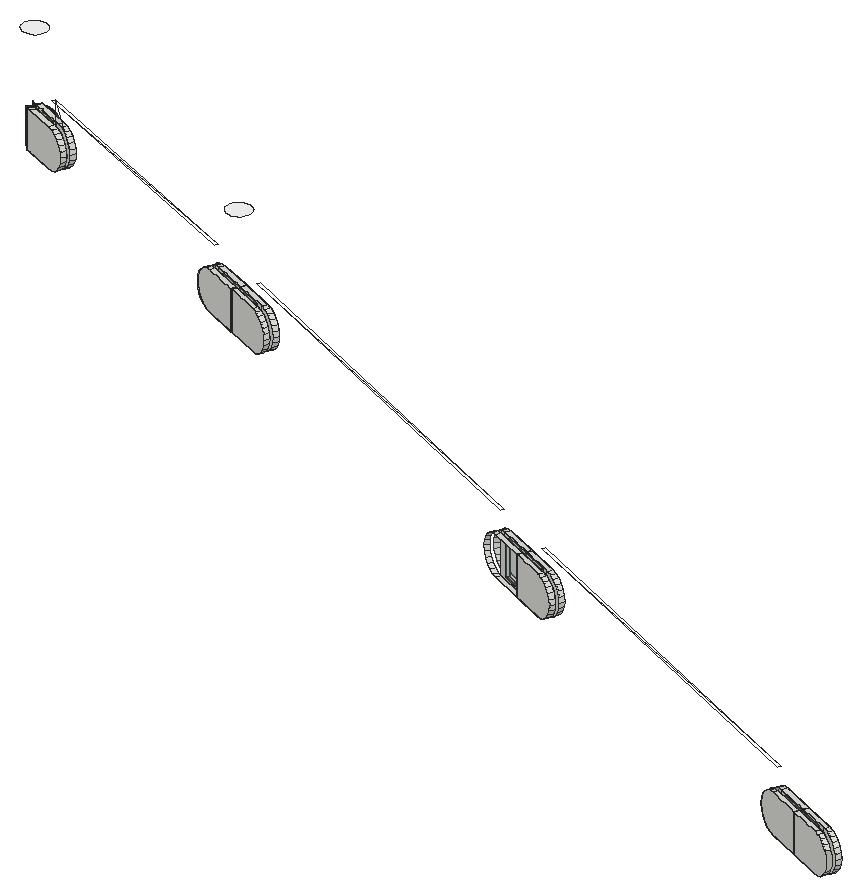
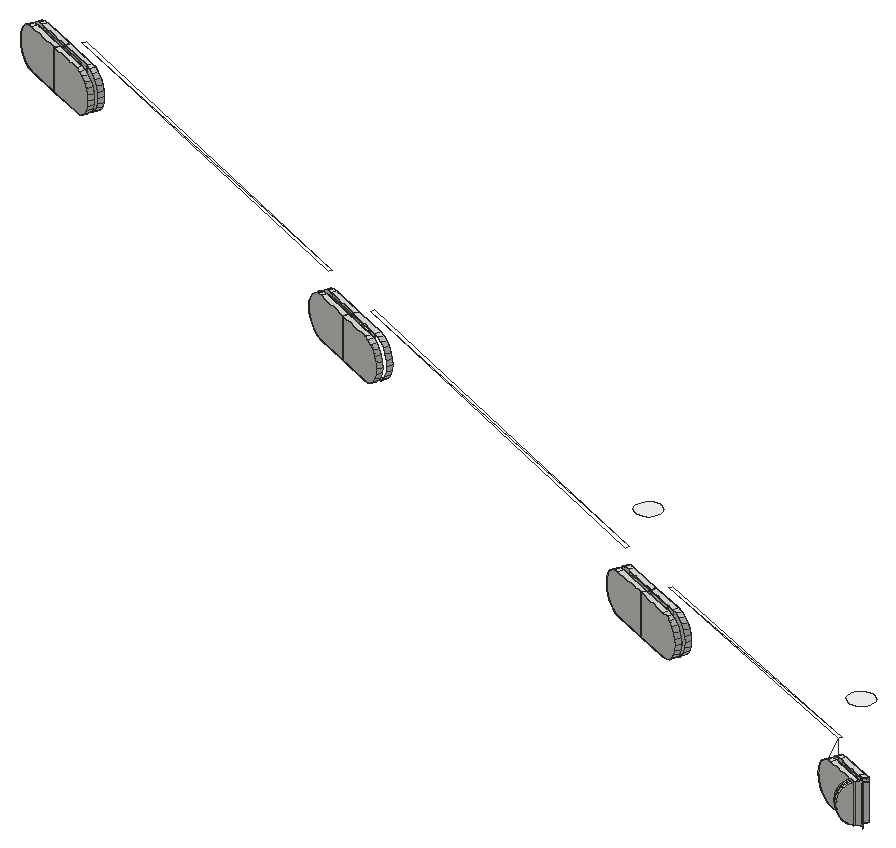
# SketchUp Ruby script. Lengths in inches.
U = 1.inch
M = Sketchup.active_model
def pt(a) = Geom::Point3d.new(a.map { |v| v * U })
def face(e, loops, mat)
  f = e.add_face(loops[0].map { |a| pt(a) })
  loops[1..].each { |l| e.add_face(l.map { |a| pt(a) }).erase! }
  f.material = f.back_material = mat if mat
  f
end
# faces: each face lists its corners as indices into pts; further lists are holes
def faces(e, pts, list, mat = nil) = list.each { |f| face(e, (f[0].is_a?(Array) ? f : [f]).map { |l| l.map { |i| pts[i] } }, mat) }
# xy, xz, yz: faces in a plane at the given z, y or x. An outline is a flat list of corners, or four numbers for a rectangle; further outlines are holes
def ring(l) = l.size == 4 ? [[l[0], l[1]], [l[2], l[1]], [l[2], l[3]], [l[0], l[3]]] : l.each_slice(2).to_a
def flat(e, list, mat, &to3) = list.each { |f| face(e, (f[0].is_a?(Array) ? f : [f]).map { |l| ring(l).map { |u, v| to3.(u, v) } }, mat) }
def xy(e, z, list, mat = nil) = flat(e, list, mat) { |x, y| [x, y, z] }
def xz(e, y, list, mat = nil) = flat(e, list, mat) { |x, z| [x, y, z] }
def yz(e, x, list, mat = nil) = flat(e, list, mat) { |y, z| [x, y, z] }
def lines(e, pts, list) = list.each { |a, b| e.add_line(pt(pts[a]), pt(pts[b])) }
# prism: a flat outline (further loops are holes) pulled along v
def prism(e, loops, v, mat = nil)
  f = face(e, loops, mat); d = Geom::Vector3d.new(v.map { |x| x * U })
  f.pushpull(f.normal.samedirection?(d) ? d.length : -d.length)
end
def box(e, o, s, mat = nil) = prism(e, [[o, [o[0] + s[0], o[1], o[2]], [o[0] + s[0], o[1] + s[1], o[2]], [o[0], o[1] + s[1], o[2]]]], [0, 0, s[2]], mat)
def at(x, y, z, deg = 0) = Geom::Transformation.translation(pt([x, y, z])) * Geom::Transformation.rotation(ORIGIN, Z_AXIS, deg.degrees)
def axes(o, x, y, z) = Geom::Transformation.new([*x, 0, *y, 0, *z, 0, *pt(o).to_a, 1])
def part(name) = M.definitions.add(name)
# library, detail: a bought-in or finely detailed component or shape, given as its bounding box
def library(name, o, s) = part(name).tap { |d| box(d.entities, o, s) }
def detail(e, o, s) = box(e.add_group.entities, o, s)
def put(e, d, t, mat = nil) = e.add_instance(d, t).tap { |i| i.material = mat if mat }
def group(e, t, mat = nil) = e.add_group.tap { |g| g.transformation = t; g.material = mat if mat }.entities
root = M.entities
M.materials.add("Glass_Safety_01").color = [204, 235, 244]
M.materials["Glass_Safety_01"].alpha = 0.1
M.materials.add("[Color_000]").color = [255, 255, 255]
xy(root,351.283,[[825.641,1098.417,823.836,1099.203,823.946,1099.456,825.618,1098.728,825.751,1098.67],[825.829,1098.85,825.697,1098.908,824.025,1099.637,824.135,1099.889,825.94,1099.103],[823.836,1099.203,822.031,1099.989,822.141,1100.242,823.946,1099.456],[824.025,1099.637,822.22,1100.423,822.33,1100.675,824.135,1099.889],[802.031,1108.7,800.226,1109.486,800.336,1109.739,802.003,1109.013,802.141,1108.953],
  [802.22,1109.133,802.082,1109.193,800.415,1109.919,800.525,1110.172,802.33,1109.386],[800.226,1109.486,798.421,1110.272,798.531,1110.525,800.336,1109.739],[800.415,1109.919,798.61,1110.705,798.72,1110.958,800.525,1110.172],[777.687,1119.303,775.888,1120.086,775.994,1120.341,777.663,1119.614,777.797,1119.555],[777.876,1119.736,777.742,1119.794,776.071,1120.522,776.181,1120.775,777.986,1119.989],
  [775.888,1120.086,775.885,1120.087,775.882,1120.089,775.992,1120.341,775.994,1120.341],[775.882,1120.089,774.07,1120.841,774.176,1121.095,775.992,1120.341],[776.069,1120.523,774.251,1121.277,774.357,1121.532,776.175,1120.777],[760.716,1126.381,759.144,1127.034,759.32,1127.233,759.338,1127.252,760.627,1126.717,760.822,1126.636],[760.897,1126.818,760.702,1126.899,759.079,1127.572,759.184,1127.827,761.003,1127.072],
  [759.144,1127.034,758.951,1127.114,759.145,1127.332,759.265,1127.282,759.32,1127.233],[758.951,1127.114,758.898,1127.136,758.926,1127.204,759.068,1127.364,759.145,1127.332],[758.926,1127.204,759.003,1127.39,759.068,1127.364],[759.32,1127.233,759.265,1127.282,759.338,1127.252],[759.338,1127.252,759.265,1127.282,759.173,1127.364,759.195,1127.388,759.342,1127.257],
  [759.265,1127.282,759.145,1127.332,759.173,1127.364]])
xy(root,351.362,[[825.39,1098.827,823.946,1099.456,824.025,1099.637,825.469,1099.008],[823.946,1099.456,822.502,1100.085,822.581,1100.265,824.025,1099.637],[801.78,1109.11,800.336,1109.739,800.415,1109.919,801.859,1109.291],[800.336,1109.739,798.892,1110.368,798.971,1110.548,800.415,1109.919],[777.436,1119.713,775.994,1120.341,776.032,1120.432,776.071,1120.522,777.515,1119.893],
  [775.992,1120.341,774.539,1120.944,774.615,1121.126,776.069,1120.523,776.032,1120.432],[775.992,1120.341,776.032,1120.432,775.994,1120.341],[760.458,1126.787,759.068,1127.364,759.115,1127.416,759.041,1127.481,759.079,1127.572,760.533,1126.969],[758.875,1127.146,758.728,1127.277,758.968,1127.547,759.041,1127.481,759.003,1127.39,759.068,1127.364],[759.068,1127.364,759.003,1127.39,759.041,1127.481,759.115,1127.416]],"Glass_Safety_01")
xy(root,353.33,[[825.39,1098.827,825.469,1099.008,824.025,1099.637,823.946,1099.456],[823.946,1099.456,824.025,1099.637,822.581,1100.265,822.502,1100.085],[801.78,1109.11,801.859,1109.291,800.415,1109.919,800.336,1109.739],[800.336,1109.739,800.415,1109.919,798.971,1110.548,798.892,1110.368],[777.436,1119.713,777.515,1119.893,776.071,1120.522,776.032,1120.432,775.994,1120.341],
  [775.992,1120.341,776.032,1120.432,776.069,1120.523,774.615,1121.126,774.539,1120.944],[775.992,1120.341,775.994,1120.341,776.032,1120.432],[760.458,1126.787,760.533,1126.969,759.079,1127.572,759.041,1127.481,759.115,1127.416,759.068,1127.364],[758.875,1127.146,759.068,1127.364,759.003,1127.39,759.041,1127.481,758.968,1127.547,758.728,1127.277],[759.068,1127.364,759.115,1127.416,759.041,1127.481,759.003,1127.39]],"Glass_Safety_01")
xy(root,353.409,[[825.641,1098.417,825.751,1098.67,825.618,1098.728,823.946,1099.456,823.836,1099.203],[825.829,1098.85,825.94,1099.103,824.135,1099.889,824.025,1099.637,825.697,1098.908],[823.836,1099.203,823.946,1099.456,822.141,1100.242,822.031,1099.989],[824.025,1099.637,824.135,1099.889,822.33,1100.675,822.22,1100.423],[802.031,1108.7,802.141,1108.953,802.003,1109.013,800.336,1109.739,800.226,1109.486],
  [802.22,1109.133,802.33,1109.386,800.525,1110.172,800.415,1109.919,802.082,1109.193],[800.226,1109.486,800.336,1109.739,798.531,1110.525,798.421,1110.272],[800.415,1109.919,800.525,1110.172,798.72,1110.958,798.61,1110.705],[777.687,1119.303,777.797,1119.555,777.663,1119.614,775.994,1120.341,775.888,1120.086],[777.876,1119.736,777.986,1119.989,776.181,1120.775,776.071,1120.522,777.742,1119.794],
  [775.888,1120.086,775.994,1120.341,775.992,1120.341,775.882,1120.089,775.885,1120.087],[775.882,1120.089,775.992,1120.341,774.176,1121.095,774.07,1120.841],[776.069,1120.523,776.175,1120.777,774.357,1121.532,774.251,1121.277],[760.716,1126.381,760.822,1126.636,760.627,1126.717,759.338,1127.252,759.32,1127.233,759.144,1127.034],[760.897,1126.818,761.003,1127.072,759.184,1127.827,759.079,1127.572,760.702,1126.899],
  [759.144,1127.034,759.32,1127.233,759.265,1127.282,759.145,1127.332,758.951,1127.114],[758.951,1127.114,759.145,1127.332,759.068,1127.364,758.926,1127.204,758.898,1127.136],[758.926,1127.204,759.068,1127.364,759.003,1127.39],[759.32,1127.233,759.338,1127.252,759.265,1127.282],[759.338,1127.252,759.342,1127.257,759.195,1127.388,759.173,1127.364,759.265,1127.282],
  [759.265,1127.282,759.173,1127.364,759.145,1127.332]])
xy(root,354.511,[[822.141,1100.242,822.22,1100.423,802.003,1109.013],[822.22,1100.423,802.082,1109.193,802.003,1109.013],[798.531,1110.525,798.61,1110.705,777.663,1119.614],[798.61,1110.705,777.742,1119.794,777.663,1119.614],[774.176,1121.095,774.251,1121.277,760.627,1126.717],
  [774.251,1121.277,760.702,1126.899,760.627,1126.717]],"Glass_Safety_01")
xy(root,357.267,[[776.077,1119.803,776.238,1119.836,776.385,1119.91,776.508,1120.019,776.598,1120.156,776.65,1120.3125,776.66,1120.477,776.627,1120.638,776.553,1120.785,776.444,1120.908,776.307,1120.998,776.151,1121.05,775.987,1121.06,775.825,1121.027,775.678,1120.953,775.555,1120.844,775.465,1120.707,775.413,1120.551,775.403,1120.387,775.436,1120.226,775.51,1120.078,775.619,1119.956,775.756,1119.865,775.912,1119.813],[759.086,1126.853,759.247,1126.886,759.394,1126.96,759.517,1127.069,759.608,1127.206,759.66,1127.362,759.669,1127.526,759.636,1127.6875,759.563,1127.834,759.454,1127.957,759.316,1128.048,759.16,1128.1,758.996,1128.11,758.835,1128.077,758.688,1128.003,758.565,1127.894,758.474,1127.756,758.423,1127.6,758.413,1127.436,758.446,1127.275,758.519,1127.128,758.629,1127.005,758.766,1126.915,758.922,1126.863]],"[Color_000]")
xz(root,1120.341,[[775.992,351.283,775.994,351.362],[775.992,351.283,775.994,353.409],[775.992,351.362,775.994,353.33],[775.992,353.33,775.994,353.409]])
p = [[825.641,1098.417,353.409],[823.836,1099.203,353.409],[823.836,1099.203,351.283],[825.641,1098.417,351.283],[825.893,1098.307,351.319],[826.128,1098.205,351.425],
  [826.33,1098.117,351.594],[826.485,1098.05,351.814],[826.582,1098.007,352.071],[826.615,1097.993,352.346],[826.582,1098.007,352.621],[826.485,1098.05,352.877],
  [826.33,1098.117,353.098],[826.128,1098.205,353.267],[825.893,1098.307,353.373],[825.751,1098.67,351.283],[825.618,1098.728,351.283],[825.618,1098.728,353.409],
  [825.751,1098.67,353.409],[826.003,1098.56,353.373],[826.238,1098.458,353.267],[826.44,1098.37,353.098],[826.595,1098.302,352.877],[826.692,1098.26,352.621],
  [826.725,1098.246,352.346],[826.692,1098.26,352.071],[826.595,1098.302,351.814],[826.44,1098.37,351.594],[826.238,1098.458,351.425],[826.003,1098.56,351.319],
  [825.829,1098.85,353.409],[825.697,1098.908,353.409],[825.697,1098.908,351.283],[825.829,1098.85,351.283],[826.082,1098.741,351.319],[826.317,1098.638,351.425],
  [826.519,1098.55,351.594],[826.674,1098.483,351.814],[826.771,1098.44,352.071],[826.804,1098.426,352.346],[826.771,1098.44,352.621],[826.674,1098.483,352.877],
  [826.519,1098.55,353.098],[826.317,1098.638,353.267],[826.082,1098.741,353.373],[826.192,1098.993,351.319],[826.427,1098.891,351.425],[823.946,1099.456,353.409],
  [823.946,1099.456,351.283],[823.946,1099.456,351.362],[825.39,1098.827,351.362],[825.39,1098.827,353.33],[823.946,1099.456,353.33],[824.135,1099.889,353.409],
  [825.94,1099.103,353.409],[826.192,1098.993,353.373],[826.427,1098.891,353.267],[826.629,1098.803,353.098],[826.784,1098.736,352.877],[826.881,1098.693,352.621],
  [826.914,1098.679,352.346],[826.881,1098.693,352.071],[826.784,1098.736,351.814],[826.629,1098.803,351.594],[825.94,1099.103,351.283],[824.135,1099.889,351.283],
  [824.025,1099.637,351.283],[824.025,1099.637,353.409],[824.025,1099.637,353.33],[825.469,1099.008,353.33],[825.469,1099.008,351.362],[824.025,1099.637,351.362],
  [822.031,1099.989,353.409],[821.779,1100.099,353.373],[821.544,1100.202,353.267],[821.342,1100.29,353.098],[821.1875,1100.357,352.877],[821.09,1100.399,352.621],
  [821.057,1100.414,352.346],[821.09,1100.399,352.071],[821.1875,1100.357,351.814],[821.342,1100.29,351.594],[821.544,1100.202,351.425],[821.779,1100.099,351.319],
  [822.031,1099.989,351.283],[822.141,1100.242,351.283],[822.141,1100.242,353.409],[822.502,1100.085,353.33],[822.502,1100.085,351.362],[822.22,1100.423,353.409],
  [822.22,1100.423,351.283],[822.581,1100.265,351.362],[822.581,1100.265,353.33],[822.33,1100.675,353.409],[822.33,1100.675,351.283],[822.078,1100.785,351.319],
  [821.843,1100.887,351.425],[821.641,1100.975,351.594],[821.486,1101.043,351.814],[821.389,1101.085,352.071],[821.355,1101.1,352.346],[821.389,1101.085,352.621],
  [821.486,1101.043,352.877],[821.641,1100.975,353.098],[821.843,1100.887,353.267],[822.078,1100.785,353.373],[821.889,1100.352,351.319],[821.654,1100.454,351.425],
  [821.889,1100.352,353.373],[821.654,1100.454,353.267],[821.452,1100.542,353.098],[821.297,1100.61,352.877],[821.2,1100.652,352.621],[821.167,1100.667,352.346],
  [821.2,1100.652,352.071],[821.297,1100.61,351.814],[821.452,1100.542,351.594],[821.968,1100.532,351.319],[821.733,1100.635,351.425],[821.531,1100.723,351.594],
  [821.376,1100.79,351.814],[821.279,1100.833,352.071],[821.245,1100.847,352.346],[821.279,1100.833,352.621],[821.376,1100.79,352.877],[821.531,1100.723,353.098],
  [821.733,1100.635,353.267],[821.968,1100.532,353.373],[802.031,1108.7,353.409],[800.226,1109.486,353.409],[800.226,1109.486,351.283],[802.031,1108.7,351.283],
  [802.283,1108.59,351.319],[802.518,1108.488,351.425],[802.72,1108.4,351.594],[802.875,1108.333,351.814],[802.972,1108.29,352.071],[803.006,1108.276,352.346],
  [802.972,1108.29,352.621],[802.875,1108.333,352.877],[802.72,1108.4,353.098],[802.518,1108.488,353.267],[802.283,1108.59,353.373],[802.141,1108.953,351.283],
  [802.003,1109.013,351.283],[802.003,1109.013,353.409],[802.141,1108.953,353.409],[802.393,1108.843,353.373],[802.628,1108.741,353.267],[802.83,1108.653,353.098],
  [802.985,1108.585,352.877],[803.082,1108.543,352.621],[803.116,1108.528,352.346],[803.082,1108.543,352.071],[802.985,1108.585,351.814],[802.83,1108.653,351.594],
  [802.628,1108.741,351.425],[802.393,1108.843,351.319],[802.22,1109.133,353.409],[802.082,1109.193,353.409],[802.082,1109.193,351.283],[802.22,1109.133,351.283],
  [802.472,1109.023,351.319],[802.707,1108.921,351.425],[802.909,1108.833,351.594],[803.064,1108.766,351.814],[803.161,1108.723,352.071],[803.194,1108.709,352.346],
  [803.161,1108.723,352.621],[803.064,1108.766,352.877],[802.909,1108.833,353.098],[802.707,1108.921,353.267],[802.472,1109.023,353.373],[802.582,1109.276,351.319],
  [802.817,1109.174,351.425],[800.336,1109.739,353.409],[800.336,1109.739,351.283],[800.336,1109.739,351.362],[801.78,1109.11,351.362],[801.78,1109.11,353.33],
  [800.336,1109.739,353.33],[800.525,1110.172,353.409],[802.33,1109.386,353.409],[802.582,1109.276,353.373],[802.817,1109.174,353.267],[803.019,1109.086,353.098],
  [803.174,1109.018,352.877],[803.271,1108.976,352.621],[803.304,1108.962,352.346],[803.271,1108.976,352.071],[803.174,1109.018,351.814],[803.019,1109.086,351.594],
  [802.33,1109.386,351.283],[800.525,1110.172,351.283],[800.415,1109.919,351.283],[800.415,1109.919,353.409],[800.415,1109.919,353.33],[801.859,1109.291,353.33],
  [801.859,1109.291,351.362],[800.415,1109.919,351.362],[798.531,1110.525,351.283],[798.531,1110.525,353.409],[798.892,1110.368,353.33],[798.892,1110.368,351.362],
  [798.61,1110.705,353.409],[798.61,1110.705,351.283],[798.971,1110.548,351.362],[798.971,1110.548,353.33],[798.72,1110.958,353.409],[798.72,1110.958,351.283],
  [798.468,1111.068,351.319],[798.233,1111.17,351.425],[798.031,1111.258,351.594],[797.876,1111.326,351.814],[797.779,1111.368,352.071],[797.746,1111.382,352.346],
  [797.779,1111.368,352.621],[797.876,1111.326,352.877],[798.031,1111.258,353.098],[798.233,1111.17,353.267],[798.468,1111.068,353.373],[798.279,1110.635,351.319],
  [798.421,1110.272,351.283],[798.169,1110.382,351.319],[798.044,1110.737,351.425],[797.934,1110.484,351.425],[798.279,1110.635,353.373],[798.044,1110.737,353.267],
  [797.842,1110.825,353.098],[797.6875,1110.892,352.877],[797.59,1110.935,352.621],[797.557,1110.949,352.346],[797.59,1110.935,352.071],[797.6875,1110.892,351.814],
  [797.842,1110.825,351.594],[798.358,1110.815,351.319],[798.123,1110.918,351.425],[797.921,1111.005,351.594],[797.766,1111.073,351.814],[797.669,1111.115,352.071],
  [797.636,1111.13,352.346],[797.669,1111.115,352.621],[797.766,1111.073,352.877],[797.921,1111.005,353.098],[798.123,1110.918,353.267],[798.358,1110.815,353.373],
  [777.687,1119.303,353.409],[775.888,1120.086,353.409],[775.888,1120.086,351.283],[777.687,1119.303,351.283],[777.939,1119.193,351.319],[778.174,1119.09,351.425],
  [778.376,1119.003,351.594],[778.531,1118.935,351.814],[778.628,1118.893,352.071],[778.662,1118.878,352.346],[778.628,1118.893,352.621],[778.531,1118.935,352.877],
  [778.376,1119.003,353.098],[778.174,1119.09,353.267],[777.939,1119.193,353.373],[777.797,1119.555,351.283],[777.663,1119.614,351.283],[777.663,1119.614,353.409],
  [777.797,1119.555,353.409],[778.049,1119.446,353.373],[778.284,1119.343,353.267],[778.486,1119.255,353.098],[778.641,1119.188,352.877],[778.738,1119.145,352.621],
  [778.772,1119.131,352.346],[778.738,1119.145,352.071],[778.641,1119.188,351.814],[778.486,1119.255,351.594],[778.284,1119.343,351.425],[778.049,1119.446,351.319],
  [777.876,1119.736,353.409],[777.742,1119.794,353.409],[777.742,1119.794,351.283],[777.876,1119.736,351.283],[778.128,1119.626,351.319],[778.363,1119.524,351.425],
  [778.565,1119.436,351.594],[778.72,1119.368,351.814],[778.817,1119.326,352.071],[778.85,1119.311,352.346],[778.817,1119.326,352.621],[778.72,1119.368,352.877],
  [778.565,1119.436,353.098],[778.363,1119.524,353.267],[778.128,1119.626,353.373],[778.238,1119.879,351.319],[778.473,1119.776,351.425],[775.994,1120.341,353.409],
  [775.994,1120.341,351.283],[775.994,1120.341,351.362],[777.436,1119.713,351.362],[777.436,1119.713,353.33],[775.994,1120.341,353.33],[776.181,1120.775,353.409],
  [777.986,1119.989,353.409],[778.238,1119.879,353.373],[778.473,1119.776,353.267],[778.675,1119.688,353.098],[778.83,1119.621,352.877],[778.927,1119.579,352.621],
  [778.96,1119.564,352.346],[778.927,1119.579,352.071],[778.83,1119.621,351.814],[778.675,1119.688,351.594],[777.986,1119.989,351.283],[776.181,1120.775,351.283],
  [776.071,1120.522,351.283],[776.071,1120.522,353.409],[776.071,1120.522,353.33],[777.515,1119.893,353.33],[777.515,1119.893,351.362],[776.071,1120.522,351.362],
  [775.885,1120.087,353.409],[775.882,1120.089,353.409],[774.07,1120.841,353.409],[773.816,1120.946,353.373],[773.579,1121.044,353.267],[773.376,1121.129,353.098],
  [773.22,1121.193,352.877],[773.122,1121.234,352.621],[773.088,1121.248,352.346],[773.122,1121.234,352.071],[773.22,1121.193,351.814],[773.376,1121.129,351.594],
  [773.579,1121.044,351.425],[773.816,1120.946,351.319],[774.07,1120.841,351.283],[775.882,1120.089,351.283],[775.885,1120.087,351.283],[775.992,1120.341,351.362],
  [775.992,1120.341,351.283],[775.992,1120.341,353.409],[775.992,1120.341,353.33],[774.539,1120.944,353.33],[774.539,1120.944,351.362],[774.176,1121.095,351.283],
  [774.176,1121.095,353.409],[776.069,1120.523,353.409],[774.251,1121.277,353.409],[774.251,1121.277,351.283],[776.069,1120.523,351.283],[776.069,1120.523,351.362],
  [774.615,1121.126,351.362],[774.615,1121.126,353.33],[776.069,1120.523,353.33],[776.175,1120.777,351.283],[776.175,1120.777,353.409],[774.357,1121.532,353.409],
  [774.357,1121.532,351.283],[774.103,1121.637,351.319],[773.866,1121.735,351.425],[773.662,1121.82,351.594],[773.506,1121.884,351.814],[773.408,1121.925,352.071],
  [773.375,1121.939,352.346],[773.408,1121.925,352.621],[773.506,1121.884,352.877],[773.662,1121.82,353.098],[773.866,1121.735,353.267],[774.103,1121.637,353.373],
  [773.922,1121.201,351.319],[773.685,1121.299,351.425],[773.922,1121.201,353.373],[773.685,1121.299,353.267],[773.481,1121.383,353.098],[773.325,1121.448,352.877],
  [773.227,1121.489,352.621],[773.194,1121.503,352.346],[773.227,1121.489,352.071],[773.325,1121.448,351.814],[773.481,1121.383,351.594],[773.997,1121.382,351.319],
  [773.76,1121.481,351.425],[773.557,1121.565,351.594],[773.401,1121.63,351.814],[773.303,1121.67,352.071],[773.269,1121.684,352.346],[773.303,1121.67,352.621],
  [773.401,1121.63,352.877],[773.557,1121.565,353.098],[773.76,1121.481,353.267],[773.997,1121.382,353.373],[758.951,1127.114,353.409],[758.898,1127.136,353.409],
  [758.898,1127.136,351.283],[758.951,1127.114,351.283],[759.144,1127.034,351.283],[760.716,1126.381,351.283],[760.97,1126.276,351.319],[761.207,1126.178,351.425],
  [761.41,1126.093,351.594],[761.566,1126.029,351.814],[761.664,1125.988,352.071],[761.698,1125.974,352.346],[761.664,1125.988,352.621],[761.566,1126.029,352.877],
  [761.41,1126.093,353.098],[761.207,1126.178,353.267],[760.97,1126.276,353.373],[760.716,1126.381,353.409],[759.144,1127.034,353.409],[760.822,1126.636,351.283],
  [760.627,1126.717,351.283],[760.627,1126.717,353.409],[760.822,1126.636,353.409],[761.076,1126.531,353.373],[761.3125,1126.432,353.267],[761.516,1126.348,353.098],
  [761.672,1126.283,352.877],[761.77,1126.243,352.621],[761.803,1126.229,352.346],[761.77,1126.243,352.071],[761.672,1126.283,351.814],[761.516,1126.348,351.594],
  [761.3125,1126.432,351.425],[761.076,1126.531,351.319],[761.848,1126.423,352.599],[761.508,1126.564,353.167],[761.388,1126.614,353.267],[761.151,1126.712,353.373],
  [760.897,1126.818,353.409],[760.702,1126.899,353.409],[760.702,1126.899,351.283],[760.897,1126.818,351.283],[761.151,1126.712,351.319],[761.388,1126.614,351.425],
  [761.591,1126.53,351.594],[761.747,1126.465,351.814],[761.845,1126.424,352.071],[761.879,1126.41,352.346],[761.257,1126.967,351.319],[761.494,1126.869,351.425],
  [759.338,1127.252,353.409],[759.338,1127.252,351.283],[759.265,1127.282,351.283],[759.145,1127.332,351.283],[759.068,1127.364,351.283],[759.003,1127.39,351.283],
  [759.003,1127.39,351.362],[759.068,1127.364,351.362],[760.458,1126.787,351.362],[760.458,1126.787,353.33],[759.068,1127.364,353.33],[759.003,1127.39,353.33],
  [759.003,1127.39,353.409],[759.068,1127.364,353.409],[759.145,1127.332,353.409],[759.265,1127.282,353.409],[759.184,1127.827,353.409],[761.003,1127.072,353.409],
  [761.257,1126.967,353.373],[761.494,1126.869,353.267],[761.697,1126.784,353.098],[761.853,1126.72,352.877],[761.951,1126.679,352.621],[761.984,1126.665,352.346],
  [761.951,1126.679,352.071],[761.853,1126.72,351.814],[761.697,1126.784,351.594],[761.003,1127.072,351.283],[759.184,1127.827,351.283],[759.079,1127.572,351.283],
  [759.079,1127.572,353.409],[759.079,1127.572,353.33],[760.533,1126.969,353.33],[760.533,1126.969,351.362],[759.079,1127.572,351.362],[758.926,1127.204,351.283],
  [758.926,1127.204,353.409],[759.115,1127.416,351.283],[759.115,1127.416,351.362],[759.115,1127.416,353.33],[759.115,1127.416,353.409],[759.173,1127.364,353.409],
  [759.32,1127.233,353.409],[759.32,1127.233,351.283],[759.173,1127.364,351.283],[759.342,1127.257,353.409],[759.525,1127.463,353.373],[759.696,1127.654,353.267],
  [759.842,1127.819,353.098],[759.954,1127.945,352.877],[760.025,1128.024,352.621],[760.049,1128.051,352.346],[760.025,1128.024,352.071],[759.954,1127.945,351.814],
  [759.842,1127.819,351.594],[759.696,1127.654,351.425],[759.525,1127.463,351.319],[759.342,1127.257,351.283],[759.378,1127.594,351.319],[759.195,1127.388,351.283],
  [758.989,1127.571,351.283],[759.172,1127.777,351.319],[759.319,1127.646,351.319],[759.136,1127.44,351.283],[758.968,1127.547,351.362],[758.968,1127.547,351.283],
  [758.762,1127.73,351.283],[758.762,1127.73,353.409],[758.968,1127.547,353.409],[758.968,1127.547,353.33],[758.989,1127.571,353.409],[759.172,1127.777,353.373],
  [759.343,1127.968,353.267],[759.489,1128.133,353.098],[759.602,1128.259,352.877],[759.672,1128.338,352.621],[759.696,1128.365,352.346],[759.672,1128.338,352.071],
  [759.602,1128.259,351.814],[759.489,1128.133,351.594],[759.343,1127.968,351.425],[759.549,1127.785,351.425],[759.49,1127.837,351.425],[797.732,1110.572,351.594],
  [776.032,1120.432,351.362],[776.032,1120.432,353.33],[758.875,1127.146,353.33],[758.875,1127.146,351.362],[758.728,1127.277,351.362],[758.728,1127.277,353.33],
  [759.041,1127.481,353.33],[759.041,1127.481,351.362],[759.695,1127.949,351.594],[759.636,1128.002,351.594],[797.577,1110.64,351.814],[759.807,1128.076,351.814],
  [759.749,1128.128,351.814],[797.48,1110.682,352.071],[759.878,1128.155,352.071],[759.819,1128.207,352.071],[797.447,1110.697,352.346],[759.902,1128.182,352.346],
  [759.843,1128.234,352.346],[797.48,1110.682,352.621],[761.845,1126.424,352.621],[759.878,1128.155,352.621],[759.819,1128.207,352.621],[797.577,1110.64,352.877],
  [761.747,1126.465,352.877],[761.591,1126.53,353.098],[759.807,1128.076,352.877],[759.749,1128.128,352.877],[797.732,1110.572,353.098],[759.695,1127.949,353.098],
  [759.636,1128.002,353.098],[797.934,1110.484,353.267],[759.549,1127.785,353.267],[759.49,1127.837,353.267],[760.702,1126.899,354.511],[798.169,1110.382,353.373],
  [759.378,1127.594,353.373],[759.319,1127.646,353.373],[798.421,1110.272,353.409],[759.195,1127.388,353.409]]
faces(root,p,[[0,1,2,3,4,5,6,7,8,9,10,11,12,13,14],[15,16,17,18,19,20,21,22,23,24,25,26,27,28,29],[29,28,5,4],[15,29,4,3],[30,31,32,33,34,35,36,37,38,39,40,41,42,43,44],[35,34,45,46],[47,17,16,48,49,50,51,52],[53,54,55,56,57,58,59,60,61,62,63,46,45,64,65],
  [34,33,64,45],[66,32,31,67,68,69,70,71],[1,72,73,74,75,76,77,78,79,80,81,82,83,84,2],[49,48,2,1,47,52],[48,85,86,47,52,87,88,49],[67,89,90,66,71,91,92,68],[66,71,68,67,53,65],[93,53,65,94,95,96,97,98,99,100,101,102,103,104,105],
  [106,85,84,83],[107,106,83,82],[90,117,95,94],[117,118,96,95],[128,129,130,131,132,133,134,135,136,137,138,139,140,141,142],[143,144,145,146,147,148,149,150,151,152,153,154,155,156,157],[157,156,133,132],[143,157,132,131],
  [158,159,160,161,162,163,164,165,166,167,168,169,170,171,172],[163,162,173,174],[175,145,144,176,177,178,179,180],[181,182,183,184,185,186,187,188,189,190,191,174,173,192,193],[162,161,192,173],[194,160,159,195,196,197,198,199],[177,176,130,129,175,180],[176,200,201,175,180,202,203,177],
  [195,204,205,194,199,206,207,196],[194,199,196,195,181,193],[208,181,193,209,210,211,212,213,214,215,216,217,218,219,220],[221,200,222,223],[224,221,223,225],[205,235,210,209],[235,236,211,210],[246,247,248,249,250,251,252,253,254,255,256,257,258,259,260],
  [261,262,263,264,265,266,267,268,269,270,271,272,273,274,275],[275,274,251,250],[261,275,250,249],[276,277,278,279,280,281,282,283,284,285,286,287,288,289,290],[281,280,291,292],[293,263,262,294,295,296,297,298],[299,300,301,302,303,304,305,306,307,308,309,292,291,310,311],[280,279,310,291],
  [312,278,277,313,314,315,316,317],[247,318,319,320,321,322,323,324,325,326,327,328,329,330,331,332,333,334,248],[334,248,247,318,319,333],[294,295,298,293,247,248],[335,336,333,319,337,338],[337,338,339,340,335,336,341,342],[343,344,345,346,347,348,349,350],[312,317,314,313,299,311],
  [347,346,351,352,343,350],[353,352,351,354,355,356,357,358,359,360,361,362,363,364,365],[366,341,332,331],[367,366,331,330],[345,377,355,354],[377,378,356,355],[388,389,390,391,392,393,394,395,396,397,398,399,400,401,402,403,404,405,406],[407,408,409,410,411,412,413,414,415,416,417,418,419,420,421],
  [421,420,395,394],[407,421,394,393],[431,430,436,437],[438,409,408,439,440,441,442,443,444,445,446,447,448,449,450,451,452,453],[454,455,456,457,458,459,460,461,462,463,464,437,436,465,466],[430,429,465,436],[467,428,427,468,469,470,471,472],[444,443,473,390,389,474,450,449],
  [475,476,477,478,479,453,480,481,440,482],[439,481,480,438,483,484,485,486,487,488,489,490,491,492,493,494,495],[494,496,497,495],[498,499,500,501],[497,501,500,496],[502,503,504,505,506,507],[498,503,502,507,506,508,509,510,511,512,513,514,515,516,517,518,499],[493,519,496,494],
  [467,472,469,468,454,466],[499,518,520,500],[496,500,520,519],[28,27,6,5],[36,35,46,63],[116,107,82,81],[118,119,97,96],[156,155,134,133],
  [164,163,174,191],[234,224,225,521],[236,237,212,211],[274,273,252,251],[282,281,292,309],[338,335,340,339],[376,367,330,329],[378,379,357,356],
  [420,419,396,395],[432,431,437,464],[492,530,519,493],[518,517,531,520],[519,520,531,530],[27,26,7,6],[37,36,63,62],[115,116,81,80],
  [119,120,98,97],[155,154,135,134],[165,164,191,190],[233,234,521,532],[237,238,213,212],[273,272,253,252],[283,282,309,308],[375,376,329,328],
  [379,380,358,357],[419,418,397,396],[433,432,464,463],[491,533,530,492],[530,531,534,533],[517,516,534,531],[38,37,62,61],[114,115,80,79],
  [120,121,99,98],[154,153,136,135],[166,165,190,189],[232,233,532,535],[238,239,214,213],[272,271,254,253],[284,283,308,307],[374,375,328,327],
  [380,381,359,358],[418,417,398,397],[434,433,463,462],[490,536,533,491],[516,515,537,534],[533,534,537,536],[39,38,61,60],[113,114,79,78],
  [121,122,100,99],[153,152,137,136],[167,166,189,188],[231,232,535,538],[239,240,215,214],[271,270,255,254],[285,284,307,306],[373,374,327,326],
  [381,382,360,359],[417,416,399,398],[435,434,462,461],[489,539,536,490],[515,514,540,537],[536,537,540,539],[40,39,60,59],[112,113,78,77],
  [122,123,101,100],[152,151,138,137],[168,167,188,187],[230,231,538,541],[240,241,216,215],[270,269,256,255],[286,285,306,305],[372,373,326,325],
  [382,383,361,360],[416,415,400,399],[542,422,435,461,460],[488,543,539,489],[514,513,544,540],[539,540,544,543],[41,40,59,58],[111,112,77,76],
  [123,124,102,101],[151,150,139,138],[169,168,187,186],[229,230,541,545],[241,242,217,216],[269,268,257,256],[287,286,305,304],[371,372,325,324],
  [383,384,362,361],[415,414,401,400],[422,542,546,547,423],[546,542,460,459],[487,548,543,488],[513,512,549,544],[543,544,549,548],[22,21,12,11],
  [42,41,58,57],[110,111,76,75],[124,125,103,102],[150,149,140,139],[170,169,186,185],[228,229,545,550],[242,243,218,217],[268,267,258,257],
  [288,287,304,303],[370,371,324,323],[384,385,363,362],[414,413,402,401],[547,546,459,458],[486,551,548,487],[548,549,552,551],[512,511,552,549],
  [21,20,13,12],[43,42,57,56],[109,110,75,74],[125,126,104,103],[149,148,141,140],[171,170,185,184],[227,228,550,553],[243,244,219,218],
  [267,266,259,258],[289,288,303,302],[369,370,323,322],[385,386,364,363],[413,412,403,402],[424,423,547,458,457],[485,554,551,486],[511,510,555,552],
  [551,552,555,554],[20,19,14,13],[44,43,56,55],[108,109,74,73],[126,127,105,104],[148,147,142,141],[172,171,184,183],[226,227,553,557],
  [244,245,220,219],[266,265,260,259],[290,289,302,301],[368,369,322,321],[386,387,365,364],[412,411,404,403],[425,424,457,456],[484,558,554,485],
  [510,509,559,555],[554,555,559,558],[19,18,0,14],[30,44,55,54],[86,108,73,72],[127,89,93,105],[147,146,128,142],[158,172,183,182],
  [201,226,557,560],[245,204,208,220],[265,264,246,260],[276,290,301,300],[342,368,321,320],[387,344,353,365],[411,410,405,404],[426,425,456,455],
  [558,561,483,484],[508,561,558,559,509]])
faces(root,p,[[85,86,108,109,110,111,112,113,114,115,116,107,106],[89,90,117,118,119,120,121,122,123,124,125,126,127],[200,201,226,227,228,229,230,231,232,233,234,224,221],[204,205,235,236,237,238,239,240,241,242,243,244,245],[341,342,368,369,370,371,372,373,374,375,376,367,366],[344,345,377,378,379,380,381,382,383,384,385,386,387],[422,423,424,425,426,427,428,429,430,431,432,433,434,435],[52,51,50,49],
  [51,50,70,69],[69,68,71,70],[87,52,49,88],[52,68,71,49],[68,92,91,71],[92,91,88,87],[180,179,178,177],[179,178,198,197],
  [197,196,199,198],[202,180,177,203],[180,196,199,177],[196,207,206,199],[207,206,203,202],[298,297,296,295],[297,296,316,315],[315,314,317,316],
  [522,523,298,295],[338,523,522,335],[317,522,523,314],[523,522,347,350],[350,349,348,347],[348,340,339,349],[449,448,447,446,445,444],[447,446,471,470],
  [470,469,472,471],[524,525,526,527],[524,448,477,476,445,525],[502,526,527,507],[449,528,529,444],[529,528,477,476],[528,529,502,507],[472,529,528,469],
  [556,423,424,425,426,427]],"Glass_Safety_01")
lines(root,p,[[478,451],[442,475]])
